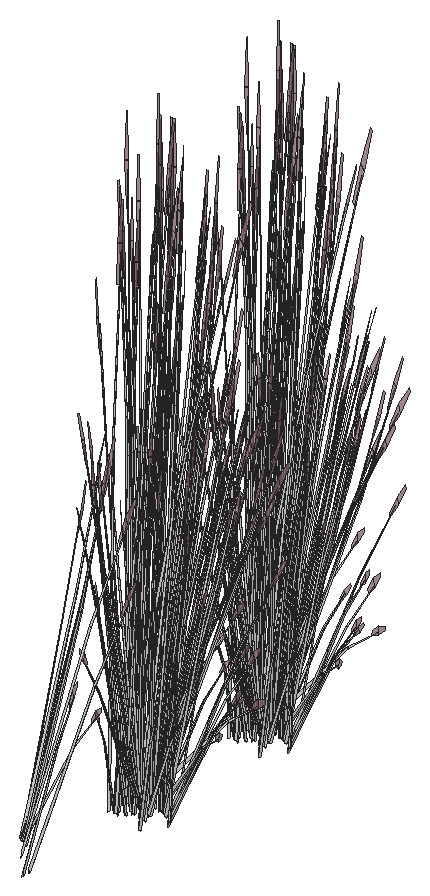
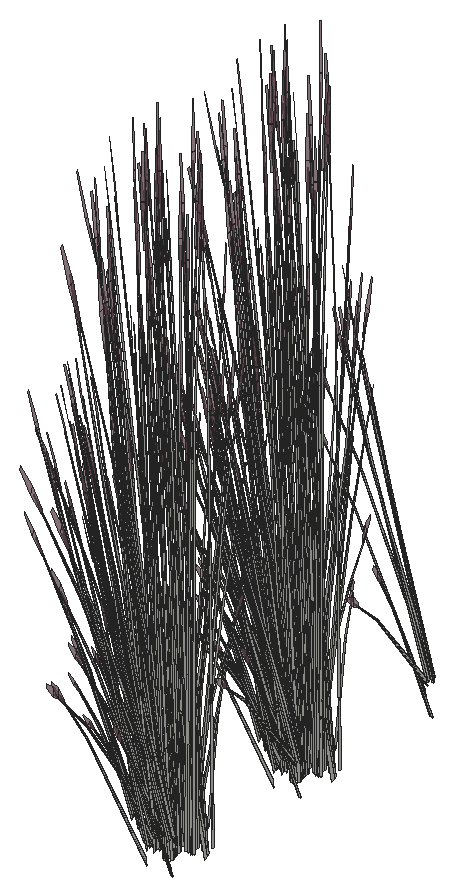
# SketchUp Ruby script. Lengths in inches.
U = 1.inch
M = Sketchup.active_model
def pt(a) = Geom::Point3d.new(a.map { |v| v * U })
def face(e, loops, mat)
  f = e.add_face(loops[0].map { |a| pt(a) })
  loops[1..].each { |l| e.add_face(l.map { |a| pt(a) }).erase! }
  f.material = f.back_material = mat if mat
  f
end
# faces: each face lists its corners as indices into pts; further lists are holes
def faces(e, pts, list, mat = nil) = list.each { |f| face(e, (f[0].is_a?(Array) ? f : [f]).map { |l| l.map { |i| pts[i] } }, mat) }
# xy, xz, yz: faces in a plane at the given z, y or x. An outline is a flat list of corners, or four numbers for a rectangle; further outlines are holes
def ring(l) = l.size == 4 ? [[l[0], l[1]], [l[2], l[1]], [l[2], l[3]], [l[0], l[3]]] : l.each_slice(2).to_a
def flat(e, list, mat, &to3) = list.each { |f| face(e, (f[0].is_a?(Array) ? f : [f]).map { |l| ring(l).map { |u, v| to3.(u, v) } }, mat) }
def xy(e, z, list, mat = nil) = flat(e, list, mat) { |x, y| [x, y, z] }
def xz(e, y, list, mat = nil) = flat(e, list, mat) { |x, z| [x, y, z] }
def yz(e, x, list, mat = nil) = flat(e, list, mat) { |y, z| [x, y, z] }
def lines(e, pts, list) = list.each { |a, b| e.add_line(pt(pts[a]), pt(pts[b])) }
# prism: a flat outline (further loops are holes) pulled along v
def prism(e, loops, v, mat = nil)
  f = face(e, loops, mat); d = Geom::Vector3d.new(v.map { |x| x * U })
  f.pushpull(f.normal.samedirection?(d) ? d.length : -d.length)
end
def box(e, o, s, mat = nil) = prism(e, [[o, [o[0] + s[0], o[1], o[2]], [o[0] + s[0], o[1] + s[1], o[2]], [o[0], o[1] + s[1], o[2]]]], [0, 0, s[2]], mat)
def at(x, y, z, deg = 0) = Geom::Transformation.translation(pt([x, y, z])) * Geom::Transformation.rotation(ORIGIN, Z_AXIS, deg.degrees)
def axes(o, x, y, z) = Geom::Transformation.new([*x, 0, *y, 0, *z, 0, *pt(o).to_a, 1])
def part(name) = M.definitions.add(name)
# library, detail: a bought-in or finely detailed component or shape, given as its bounding box
def library(name, o, s) = part(name).tap { |d| box(d.entities, o, s) }
def detail(e, o, s) = box(e.add_group.entities, o, s)
def put(e, d, t, mat = nil) = e.add_instance(d, t).tap { |i| i.material = mat if mat }
def group(e, t, mat = nil) = e.add_group.tap { |g| g.transformation = t; g.material = mat if mat }.entities
root = M.entities
M.materials.add("LightPink_Translucent").color = [144, 107, 117]
M.materials["LightPink_Translucent"].alpha = 0.75
c1 = part("blade")
p = [[2.15,0.21,22],[0,0.17,0],[0.09,0.45,0],[2.18,0.31,22],[2.29,0.31,22],[0.38,0.45,0],
  [2.48,0.24,33],[2.49,0.24,33],[2.48,0.22,33]]
faces(c1.entities,p,[[0,1,2,3],[4,5,2,3],[6,3,4,7],[8,0,3,6]])
c2 = part("seeds")
p = [[0.3,-0.1,1.38],[-0.01,-0.03,1.59],[-0.01,-0.03,0.03],[0.14,-0.07,-0.07],[0.29,-0.03,3],[0.15,0.01,3.11]]
faces(c2.entities,p,[[0,1,2,3],[1,0,4,5]],"LightPink_Translucent")
c3 = part("blade with seeds")
put(c3.entities,c1,at(0,0,0))
put(c3.entities,c2,axes([2.4,0.25,30.99],[1.5799,-0.05474,1.17369],[-0.12525,1.92788,0.29478],[-0.07173,-0.02425,1.56792]))
put(root,c3,axes([342.66,137.39,656.125],[0.00872,-0.13732,1.17261],[0.41669,-0.15339,-0.25218],[0.12863,0.16436,0.50135]))
put(root,c3,axes([341.53,137.87,658.13],[0.48353,-0.19287,-0.09971],[0.23761,0.34232,-0.55346],[0.0638,0.14425,0.84097]))
put(root,c3,axes([341.61,137.95,655.22],[0.07997,-0.02254,1.44601],[0.48102,0.12407,-0.2209],[0.01407,0.13984,0.2463]))
put(root,c3,axes([341.94,137.86,657.84],[0.48573,0.10385,-0.41901],[-0.16649,0.35605,-0.32456],[0.04454,0.14335,0.80174]))
put(root,c3,axes([342.22,137.12,657.18],[-0.11295,-0.13301,1.40529],[0.52192,-0.11198,0.11363],[0.11796,0.20881,0.60075]))
put(root,c3,axes([341.72,138.07,657.71],[-0.14896,0.31857,-0.29039],[-0.4346,-0.09292,0.3749],[0.03985,0.12826,0.71734]))
put(root,c3,axes([341.77,137.79,658.08],[0.23583,0.33684,-0.58257],[-0.48546,0.18772,0.0703],[0.05515,0.16275,0.8241]))
put(root,c3,axes([341.41,138.64,657.87],[0.06263,0.06671,1.43454],[0.50546,0.02621,-0.22687],[0.05083,0.14712,0.11505]))
put(root,c3,axes([343.01,147.42,656.125],[-0.14045,0.08385,1.17261],[-0.42064,-0.14676,-0.25218],[0.07797,-0.18252,0.50135]))
put(root,c3,axes([343.35,148.04,658.08],[0.01286,-0.38319,-0.58257],[0.54141,0.02574,0.0703],[0.05714,-0.16234,0.8241]))
put(root,c3,axes([344.11,147.4375,657.87],[-0.00477,-0.08245,1.43454],[-0.40285,-0.23829,-0.22687],[0.06228,-0.14445,0.11505]))
put(root,c3,axes([342.74,147.84,657.18],[-0.092,0.14239,1.40529],[-0.38596,-0.29467,0.11363],[0.17411,-0.18366,0.60075]))
put(root,c3,axes([344,147.14,657.86],[-0.05018,0.03164,1.45454],[-0.49165,-0.10676,-0.13744],[-0.0178,-0.13809,0.2574]))
put(root,c3,axes([342.49,146.75,656.27],[0.06339,0.24157,0.94186],[-0.35163,-0.13379,0.69201],[0.03784,-0.12369,0.20745]))
put(root,c3,axes([343.24,147.91,657.84],[-0.35372,-0.27835,-0.41901],[0.37366,-0.24377,-0.32456],[0.05382,-0.14142,0.80174]))
put(root,c3,axes([342.47,147.5,657.88],[0.48688,0.1083,0.39362],[-0.16649,0.35605,0.32456],[-0.02926,-0.14002,0.8145]))
put(root,c3,axes([343.61,148.06,658.13],[-0.54305,-0.02053,-0.09971],[0.01484,-0.38862,-0.55346],[0.03772,-0.14967,0.84097]))
put(root,c3,axes([343.57,147.81,657.71],[0.33433,-0.21811,-0.29039],[0.31649,0.24905,0.3749],[0.04815,-0.12654,0.71734]))
put(root,c3,axes([342.6,147.47,657.88],[0.36409,-0.14079,0.05273],[0.17821,0.25674,0.41509],[-0.03516,-0.11317,0.63295]))
put(root,c3,axes([343.99,147.67,655.22],[-0.07396,-0.03263,1.44601],[-0.18997,-0.3646,-0.2209],[0.12815,-0.09894,0.2463]))
put(root,c3,axes([343.57,147.89,657.88],[0.35185,0.28265,0.39362],[-0.37366,0.24377,0.32456],[0.0649,-0.13261,0.8145]))
put(root,c3,axes([343.7,147.92,657.88],[0.40605,0.0193,0.05273],[-0.01113,0.29147,0.41509],[0.04249,-0.11165,0.63295]))
put(root,c3,axes([343.4,148.12,658.14],[-0.33433,0.21811,0.29039],[-0.31649,-0.24905,-0.3749],[0.04815,-0.12654,0.71734]))
put(root,c3,axes([343.99,148.7,658.08],[0.2581,-0.32687,-0.58257],[0.45228,0.2323,0.0703],[0.15411,-0.11843,0.8241]))
put(root,c3,axes([341.2,147.75,655.95],[-0.30893,-0.41511,0],[0.51685,-0.2315,-0.42318],[0.11772,-0.05273,1.34243]))
put(root,c3,axes([343.98,148.55,657.84],[-0.12693,-0.37826,-0.41901],[0.48071,-0.06617,-0.32456],[0.13776,-0.1016,0.80174]))
put(root,c3,axes([344.2,148.82,658.13],[-0.45707,-0.22842,-0.09971],[0.26332,-0.3308,-0.55346],[0.12913,-0.11499,0.84097]))
put(root,c3,axes([341.62,147.6875,655.65],[0.46245,-0.20713,-0.40713],[0.27641,0.37142,0],[0.10533,-0.04718,1.29153]))
put(root,c3,axes([344.36,148.4,656.125],[-0.17652,-0.01227,1.17261],[-0.18084,-0.32916,-0.25218],[0.21685,-0.09312,0.50135]))
put(root,c3,axes([345.33,148.72,657.86],[-0.06454,-0.00315,1.45454],[-0.268,-0.33712,-0.13744],[0.10763,-0.11085,0.2574]))
put(root,c3,axes([342.17,148.54,655.6875],[0.33282,-0.31137,-0.51129],[0.41344,0.28235,-0.13419],[0.13336,-0.07767,1.12859]))
put(root,c3,axes([344.57,147.8,656.27],[-0.16458,0.21088,0.94186],[-0.14146,-0.28332,0.69201],[0.13593,-0.07099,0.20745]))
put(root,c3,axes([344.33,148.59,657.71],[0.43011,-0.0592,-0.29039],[0.11357,0.33844,0.3749],[0.12326,-0.0909,0.71734]))
put(root,c3,axes([341.59,149.08,655.8125],[0.23974,-0.37328,-0.36686],[0.49814,0.17965,0.17656],[0,-0.08605,1.17788]))
put(root,c3,axes([341.81,148.9,656.1875],[-0.05758,-0.4727,-0.23858],[0.59969,-0.02858,-0.41002],[0.1056,-0.06296,1.3096]))
put(root,c3,axes([343.98,148.79,658.14],[-0.43011,0.0592,0.29039],[-0.11357,-0.33844,-0.3749],[0.12326,-0.0909,0.71734]))
put(root,c3,axes([341.73,147.85,655.66],[0.46099,0.1025,-0.25402],[-0.11607,0.36097,0.25402],[0.09293,-0.04163,1.13959]))
put(root,c3,axes([344.37,148.74,657.88],[0.33921,0.17422,0.05273],[-0.19749,0.2481,0.41509],[0.10876,-0.08021,0.63295]))
put(root,c3,axes([344.27,148.66,657.88],[0.12254,0.38127,0.39362],[-0.48071,0.06617,0.32456],[0.14168,-0.08967,0.8145]))
put(root,c3,axes([345.57,149.125,657.87],[0.06857,-0.0631,1.43454],[-0.08776,-0.38707,-0.22687],[0.17204,-0.07339,0.11505]))
put(root,c3,axes([341.88,149.27,656],[0.55674,0.20078,0.19733],[-0.26794,0.4172,0.41002],[0,-0.09617,1.31645]))
put(root,c3,axes([341.7,148.99,656.23],[-0.53657,0.02557,0.36686],[-0.04852,-0.4245,-0.17656],[0.09606,-0.04302,1.17788]))
put(root,c3,axes([344.22,149.71,658.13],[-0.24861,-0.37512,-0.09971],[0.44125,-0.18434,-0.55346],[0.18594,-0.04949,0.84097]))
put(root,c3,axes([344.2,149.39,657.84],[0.13386,-0.37682,-0.41901],[0.45895,0.12916,-0.32456],[0.18478,-0.03455,0.80174]))
put(root,c3,axes([343.47,147.86,655.95],[0.30893,-0.41511,0],[0.51685,0.2315,-0.42318],[0.11772,0.05273,1.34243]))
put(root,c3,axes([341.69,149.14,655.9375],[0.21483,0.46323,0.37519],[-0.61383,0.16108,0.14723],[0.0075,-0.08512,1.30262]))
put(root,c3,axes([344.6875,149.5,655.625],[-0.31825,0.04971,1.16098],[-0.05066,-0.39572,0.06645],[0.2229,-0.0599,0.66064]))
put(root,c3,axes([345.27,149.15,655.85],[-0.30634,-0.2649,-0.0532],[0.33551,-0.24272,-0.24121],[0.09507,-0.01709,0.7956]))
put(root,c3,axes([342.46,149.18,655.81],[0,-0.47933,0],[0.61786,0,0],[0,0,1.47154]))
put(root,c3,axes([343.21,148.07,656.03],[-0.46245,-0.20713,0.40713],[0.27641,-0.37142,0],[0.10533,0.04718,1.29153]))
put(root,c3,axes([344.11,149.53,658.08],[0.43419,-0.18296,-0.58257],[0.24197,0.37661,0.0703],[0.20979,-0.04278,0.8241]))
put(root,c3,axes([342.17,148.88,655.9375],[-0.40969,0.37595,0.37519],[-0.48673,-0.33186,0.14723],[0.09877,-0.03752,1.30262]))
put(root,c3,axes([341.45,148.26,656.03],[-0.14274,0.41171,0.14467],[-0.52234,-0.11651,0.28771],[0.09023,-0.00201,1.31534]))
put(root,c3,axes([344.05,149.6,658.14],[-0.41064,-0.11557,0.29039],[0.11977,-0.33716,-0.3749],[0.16533,-0.03092,0.71734]))
put(root,c3,axes([341.24,148.59,655.31],[-0.48636,0.16585,1.05721],[-0.1548,-0.47588,0.41079],[0.29865,0.00792,1.20246]))
put(root,c3,axes([342.54,148.72,656.15],[0.09532,-0.36971,0.11873],[0.46572,0.06418,-0.33905],[0.08476,0.03796,1.0393]))
put(root,c3,axes([345.04,149.24,655.22],[-0.02582,-0.06289,1.44601],[0.17911,-0.36789,-0.2209],[0.18067,-0.00529,0.2463]))
put(root,c3,axes([342.35,148.8125,656.23],[-0.29683,-0.34771,0.36686],[0.44961,-0.24485,-0.17656],[0.09606,0.04302,1.17788]))
put(root,c3,axes([342.5,148.84,656.1875],[0.49889,-0.27503,-0.23858],[0.33175,0.38862,-0.41002],[0.12309,0.03947,1.3096]))
put(root,c3,axes([344.48,149.5625,657.71],[0.41064,0.11557,-0.29039],[-0.11977,0.33716,0.3749],[0.16533,-0.03092,0.71734]))
put(root,c3,axes([343.75,148.11,655.65],[0.46245,0.20713,-0.40713],[-0.27641,0.37142,0],[0.10533,0.04718,1.29153]))
put(root,c3,axes([342.88,149.29,655.81],[0.55282,0,0],[0,0.42888,0],[0,0,1.46294]))
put(root,c3,axes([343.03,148.28,656.03],[-0.53096,0.10995,0.14467],[-0.13111,-0.40919,0.28771],[0.04735,0.05962,1.31534]))
put(root,c3,axes([343.36,149.14,657.18],[-0.20495,0.00938,1.40529],[0.13596,-0.40664,0.11363],[0.29207,0.02515,0.60075]))
put(root,c3,axes([343.625,148.26,655.66],[0.11607,0.36097,-0.25402],[-0.46099,0.1025,0.25402],[0.09293,0.04163,1.13959]))
put(root,c3,axes([344.42,149.7,657.88],[0.18148,0.28246,0.05273],[-0.33093,0.13825,0.41509],[0.14588,-0.02728,0.63295]))
put(root,c3,axes([342.7,149.07,655.95],[-0.62452,-0.08728,0.40343],[0.1271,-0.49295,0.15831],[0.09127,0.0476,1.40067]))
put(root,c3,axes([344.39,149.6,657.88],[-0.1396,0.37772,0.39362],[-0.45895,-0.12916,0.32456],[0.18049,-0.0227,0.8145]))
put(root,c3,axes([342.2,150.29,655.81],[-0.16122,-0.35715,0],[0.46037,-0.12507,0],[0,0,1.26584]))
put(root,c3,axes([342.8,150.24,655.79],[0.51876,-0.14056,-0.15742],[0.18228,0.40489,0.00007],[0.05726,-0.01554,1.42596]))
put(root,c3,axes([342.87,149.47,655.82],[0.34492,0.26758,0],[-0.34492,0.26758,0],[0,0,1.38798]))
put(root,c3,axes([343.8,149.35,656.03],[-0.38822,-0.30175,0.14467],[0.39123,-0.29268,0.28771],[-0.04288,0.06162,1.31534]))
put(root,c3,axes([343.08,148.9,655.6875],[0.514,0.06792,-0.51129],[-0.10846,0.41895,-0.13419],[0.15339,0.05076,1.12859]))
put(root,c3,axes([345.35,149.63,656.27],[-0.30529,0.06839,0.94186],[0.1437,-0.28265,0.69201],[0.16196,0.01934,0.20745]))
put(root,c3,axes([342.86,149.16,656.23],[0.23974,-0.37328,0.36686],[0.49814,0.17965,-0.17656],[0,0.08605,1.17788]))
put(root,c3,axes([345.21,150.83,657.86],[-0.04468,-0.03627,1.45454],[0.09773,-0.38875,-0.13744],[0.17599,-0.02484,0.2574]))
put(root,c3,axes([342.77,149.37,655.88],[0,0.4791,-0.04622],[-0.61786,0,0],[0,0.01506,1.47081]))
put(root,c3,axes([342.8125,149.03,655.8125],[0.29683,0.34771,-0.36686],[-0.44961,0.24485,0.17656],[0.09606,0.04302,1.17788]))
put(root,c3,axes([344.82,150.5,657.22],[-0.09457,-0.34824,-0.02863],[0.44699,-0.08006,-0.12982],[0.09334,0.02208,0.42819]))
put(root,c3,axes([343.66,150.49,658.13],[0.02646,-0.4213,-0.09971],[0.50094,0.01152,-0.55346],[0.19293,0.02926,0.84097]))
put(root,c3,axes([344.12,149.37,656.03],[0,-0.41426,0.40713],[0.55282,0,0],[0,0.09435,1.29153]))
put(root,c3,axes([343.07,149.24,656.15],[0.46037,-0.12081,0.11873],[0.16122,0.34498,-0.33905],[0,0.07592,1.0393]))
put(root,c3,axes([343.59,150.33,658.14],[-0.28114,-0.25937,0.29039],[0.32102,-0.24553,-0.3749],[0.16311,0.03736,0.71734]))
put(root,c3,axes([344.78,150.08,656.125],[-0.119,-0.10189,1.17261],[0.15483,-0.33705,-0.25218],[0.24077,0.04566,0.50135]))
put(root,c3,axes([342.65,150.46,655.81],[0.49814,0.18599,0],[-0.23974,0.38645,0],[0,0,1.43462]))
put(root,c3,axes([344.1,150.24,657.87],[0.106,-0.00701,1.43454],[0.29074,-0.32184,-0.22687],[0.18854,0.04248,0.11505]))
put(root,c3,axes([343.6875,150.29,658.08],[0.49394,0.00997,-0.58257],[-0.03317,0.42002,0.0703],[0.20925,0.04433,0.8241]))
put(root,c3,axes([342.47,150.3,655.88],[0.21483,0.47591,-0.0493],[-0.61383,0.16676,0],[0.0075,0.01662,1.41182]))
put(root,c3,axes([344.49,149.4375,655.95],[0.61786,0,0],[0,0.463,-0.42318],[0,0.10545,1.34243]))
put(root,c3,axes([344.25,149.67,655.8],[-0.61756,-0.00331,-0.04081],[0,-0.463,0.40953],[-0.01941,0.1054,1.29849]))
put(root,c3,axes([342.91,149.27,656.1875],[0.55647,0.19766,-0.23858],[-0.26794,0.4172,-0.41002],[0.01749,0.10243,1.3096]))
put(root,c3,axes([343.98,150.46,657.71],[0.28114,0.25937,-0.29039],[-0.32102,0.24553,0.3749],[0.16311,0.03736,0.71734]))
put(root,c3,axes([344.12,149.74,655.66],[-0.34492,0.25847,-0.25402],[-0.34492,-0.25847,0.25402],[0,0.08325,1.13959]))
put(root,c3,axes([343.84,150.5625,657.88],[-0.02488,0.31501,0.05273],[-0.3757,-0.00864,0.41509],[0.14392,0.03296,0.63295]))
put(root,c3,axes([342.85,149.58,655.8125],[-0.23974,0.37328,-0.36686],[-0.49814,-0.17965,0.17656],[0,0.08605,1.17788]))
put(root,c3,axes([343.875,150.46,657.88],[-0.36434,0.27297,0.39362],[-0.31422,-0.28988,0.32456],[0.17094,0.05035,0.8145]))
put(root,c3,axes([342.72,150.78,658.14],[-0.07631,-0.33368,0.29039],[0.43626,-0.08811,-0.3749],[0.11718,0.09562,0.71734]))
put(root,c3,axes([344.36,149.75,655.65],[0,0.41426,-0.40713],[-0.55282,0,0],[0,0.09435,1.29153]))
put(root,c3,axes([342.97,149.8,657.18],[-0.18354,-0.07137,1.40529],[0.37983,-0.29943,0.11363],[0.23673,0.13508,0.60075]))
put(root,c3,axes([343.01,148.86,657.67],[-0.42697,-0.21524,1.13392],[0.45084,-0.33512,0.48925],[0.13776,0.20196,1.09604]))
put(root,c3,axes([343.65,150.61,656.27],[-0.27821,-0.11912,0.94186],[0.35924,-0.12103,0.69201],[0.09689,0.10252,0.20745]))
put(root,c3,axes([342.68,150.95,658.13],[0.29444,-0.35459,-0.09971],[0.4264,0.20428,-0.55346],[0.14822,0.10018,0.84097]))
put(root,c3,axes([342.29,151.24,657.86],[0.00146,-0.05015,1.45454],[0.42344,-0.22127,-0.13744],[0.14708,0.07898,0.2574]))
put(root,c3,axes([343.73,151.05,655.22],[0.036,-0.05981,1.44601],[0.45322,-0.17614,-0.2209],[0.1374,0.09116,0.2463]))
put(root,c3,axes([343.13,149.69,655.72],[0.18118,0.37929,-0.56754],[-0.52191,0.1366,-0.14895],[0.02003,0.12844,1.25274]))
put(root,c3,axes([343.03,150.77,657.84],[0.48758,-0.09847,-0.41901],[0.08529,0.37293,-0.32456],[0.13096,0.10687,0.80174]))
put(root,c3,axes([341.67,150.83,658.14],[0.14896,-0.31857,0.29039],[0.4346,0.09292,-0.3749],[0.03985,0.12826,0.71734]))
put(root,c3,axes([343.7,151.15,656.1875],[-0.31686,-0.01299,0.86149],[0.20925,-0.27594,0.47565],[0.12517,0.09804,0.67577]))
put(root,c3,axes([342.79,151.08,657.88],[-0.22457,0.26316,0.05273],[-0.3198,-0.15321,0.41509],[0.10339,0.08437,0.63295]))
put(root,c3,axes([342.26,151.97,658.63],[0.34145,-0.23766,-0.0532],[0.31287,0.26029,-0.24121],[0.02203,0.07375,0.7956]))
put(root,c3,axes([342.88,151.01,657.88],[-0.49145,0.09507,0.39362],[-0.08529,-0.37293,0.32456],[0.11558,0.10991,0.8145]))
put(root,c3,axes([342.66,150.48,656.125],[0.00872,-0.13732,1.17261],[0.41669,-0.15339,-0.25218],[0.12863,0.16436,0.50135]))
put(root,c3,axes([341.53,150.96,658.13],[0.48353,-0.19287,-0.09971],[0.23761,0.34232,-0.55346],[0.0638,0.14425,0.84097]))
put(root,c3,axes([341.61,151.04,655.22],[0.07997,-0.02254,1.44601],[0.48102,0.12407,-0.2209],[0.01407,0.13984,0.2463]))
put(root,c3,axes([341.94,150.95,657.84],[0.48573,0.10385,-0.41901],[-0.16649,0.35605,-0.32456],[0.04454,0.14335,0.80174]))
put(root,c3,axes([342.22,150.21,657.18],[-0.11295,-0.13301,1.40529],[0.52192,-0.11198,0.11363],[0.11796,0.20881,0.60075]))
put(root,c3,axes([341.72,151.17,657.71],[-0.14896,0.31857,-0.29039],[-0.4346,-0.09292,0.3749],[0.03985,0.12826,0.71734]))
put(root,c3,axes([341.77,150.88,658.08],[0.23583,0.33684,-0.58257],[-0.48546,0.18772,0.0703],[0.05515,0.16275,0.8241]))
put(root,c3,axes([341.41,151.73,657.87],[0.06263,0.06671,1.43454],[0.50546,0.02621,-0.22687],[0.05083,0.14712,0.11505]))
put(root,c3,axes([343.01,160.05,656.125],[-0.14045,0.08385,1.17261],[-0.42064,-0.14676,-0.25218],[0.07797,-0.18252,0.50135]))
put(root,c3,axes([343.35,160.67,658.08],[0.01286,-0.38319,-0.58257],[0.54141,0.02574,0.0703],[0.05714,-0.16234,0.8241]))
put(root,c3,axes([344.11,160.08,657.87],[-0.00477,-0.08245,1.43454],[-0.40285,-0.23829,-0.22687],[0.06228,-0.14445,0.11505]))
put(root,c3,axes([342.41,160.06,657.71],[0.14896,-0.31857,-0.29039],[0.4346,0.09292,0.3749],[-0.03985,-0.12826,0.71734]))
put(root,c3,axes([342.74,160.48,657.18],[-0.092,0.14239,1.40529],[-0.38596,-0.29467,0.11363],[0.17411,-0.18366,0.60075]))
put(root,c3,axes([344,159.78,657.86],[-0.05018,0.03164,1.45454],[-0.49165,-0.10676,-0.13744],[-0.0178,-0.13809,0.2574]))
put(root,c3,axes([342.49,159.39,656.27],[0.06339,0.24157,0.94186],[-0.35163,-0.13379,0.69201],[0.03784,-0.12369,0.20745]))
put(root,c3,axes([343.24,160.55,657.84],[-0.35372,-0.27835,-0.41901],[0.37366,-0.24377,-0.32456],[0.05382,-0.14142,0.80174]))
put(root,c3,axes([342.47,160.13,657.88],[0.48688,0.1083,0.39362],[-0.16649,0.35605,0.32456],[-0.02926,-0.14002,0.8145]))
put(root,c3,axes([343.61,160.69,658.13],[-0.54305,-0.02053,-0.09971],[0.01484,-0.38862,-0.55346],[0.03772,-0.14967,0.84097]))
put(root,c3,axes([343.57,160.44,657.71],[0.33433,-0.21811,-0.29039],[0.31649,0.24905,0.3749],[0.04815,-0.12654,0.71734]))
put(root,c3,axes([342.6,160.11,657.88],[0.36409,-0.14079,0.05273],[0.17821,0.25674,0.41509],[-0.03516,-0.11317,0.63295]))
put(root,c3,axes([343.99,160.3125,655.22],[-0.07396,-0.03263,1.44601],[-0.18997,-0.3646,-0.2209],[0.12815,-0.09894,0.2463]))
put(root,c3,axes([343.57,160.53,657.88],[0.35185,0.28265,0.39362],[-0.37366,0.24377,0.32456],[0.0649,-0.13261,0.8145]))
put(root,c3,axes([343.7,160.56,657.88],[0.40605,0.0193,0.05273],[-0.01113,0.29147,0.41509],[0.04249,-0.11165,0.63295]))
put(root,c3,axes([343.4,160.75,658.14],[-0.33433,0.21811,0.29039],[-0.31649,-0.24905,-0.3749],[0.04815,-0.12654,0.71734]))
put(root,c3,axes([343.99,161.34,658.08],[0.2581,-0.32687,-0.58257],[0.45228,0.2323,0.0703],[0.15411,-0.11843,0.8241]))
put(root,c3,axes([341.2,160.39,655.95],[-0.30893,-0.41511,0],[0.51685,-0.2315,-0.42318],[0.11772,-0.05273,1.34243]))
put(root,c3,axes([343.98,161.1875,657.84],[-0.12693,-0.37826,-0.41901],[0.48071,-0.06617,-0.32456],[0.13776,-0.1016,0.80174]))
put(root,c3,axes([344.2,161.46,658.13],[-0.45707,-0.22842,-0.09971],[0.26332,-0.3308,-0.55346],[0.12913,-0.11499,0.84097]))
put(root,c3,axes([341.62,160.33,655.65],[0.46245,-0.20713,-0.40713],[0.27641,0.37142,0],[0.10533,-0.04718,1.29153]))
put(root,c3,axes([344.36,161.04,656.125],[-0.17652,-0.01227,1.17261],[-0.18084,-0.32916,-0.25218],[0.21685,-0.09312,0.50135]))
put(root,c3,axes([345.33,161.36,657.86],[-0.06454,-0.00315,1.45454],[-0.268,-0.33712,-0.13744],[0.10763,-0.11085,0.2574]))
put(root,c3,axes([342.17,161.17,655.6875],[0.33282,-0.31137,-0.51129],[0.41344,0.28235,-0.13419],[0.13336,-0.07767,1.12859]))
put(root,c3,axes([344.57,160.4375,656.27],[-0.16458,0.21088,0.94186],[-0.14146,-0.28332,0.69201],[0.13593,-0.07099,0.20745]))
put(root,c3,axes([344.33,161.23,657.71],[0.43011,-0.0592,-0.29039],[0.11357,0.33844,0.3749],[0.12326,-0.0909,0.71734]))
put(root,c3,axes([341.59,161.72,655.8125],[0.23974,-0.37328,-0.36686],[0.49814,0.17965,0.17656],[0,-0.08605,1.17788]))
put(root,c3,axes([341.81,161.54,656.1875],[-0.05758,-0.4727,-0.23858],[0.59969,-0.02858,-0.41002],[0.1056,-0.06296,1.3096]))
put(root,c3,axes([343.98,161.43,658.14],[-0.43011,0.0592,0.29039],[-0.11357,-0.33844,-0.3749],[0.12326,-0.0909,0.71734]))
put(root,c3,axes([341.73,160.49,655.66],[0.46099,0.1025,-0.25402],[-0.11607,0.36097,0.25402],[0.09293,-0.04163,1.13959]))
put(root,c3,axes([344.37,161.375,657.88],[0.33921,0.17422,0.05273],[-0.19749,0.2481,0.41509],[0.10876,-0.08021,0.63295]))
put(root,c3,axes([344.27,161.3,657.88],[0.12254,0.38127,0.39362],[-0.48071,0.06617,0.32456],[0.14168,-0.08967,0.8145]))
put(root,c3,axes([345.57,161.76,657.87],[0.06857,-0.0631,1.43454],[-0.08776,-0.38707,-0.22687],[0.17204,-0.07339,0.11505]))
put(root,c3,axes([341.88,161.91,656],[0.55674,0.20078,0.19733],[-0.26794,0.4172,0.41002],[0,-0.09617,1.31645]))
put(root,c3,axes([341.7,161.625,656.23],[-0.53657,0.02557,0.36686],[-0.04852,-0.4245,-0.17656],[0.09606,-0.04302,1.17788]))
put(root,c3,axes([344.22,162.35,658.13],[-0.24861,-0.37512,-0.09971],[0.44125,-0.18434,-0.55346],[0.18594,-0.04949,0.84097]))
put(root,c3,axes([344.2,162.03,657.84],[0.13386,-0.37682,-0.41901],[0.45895,0.12916,-0.32456],[0.18478,-0.03455,0.80174]))
put(root,c3,axes([343.47,160.49,655.95],[0.30893,-0.41511,0],[0.51685,0.2315,-0.42318],[0.11772,0.05273,1.34243]))
put(root,c3,axes([341.69,161.78,655.9375],[0.21483,0.46323,0.37519],[-0.61383,0.16108,0.14723],[0.0075,-0.08512,1.30262]))
put(root,c3,axes([344.6875,162.13,655.625],[-0.31825,0.04971,1.16098],[-0.05066,-0.39572,0.06645],[0.2229,-0.0599,0.66064]))
put(root,c3,axes([345.27,161.78,655.85],[-0.30634,-0.2649,-0.0532],[0.33551,-0.24272,-0.24121],[0.09507,-0.01709,0.7956]))
put(root,c3,axes([342.46,161.82,655.81],[0,-0.47933,0],[0.61786,0,0],[0,0,1.47154]))
put(root,c3,axes([343.21,160.71,656.03],[-0.46245,-0.20713,0.40713],[0.27641,-0.37142,0],[0.10533,0.04718,1.29153]))
put(root,c3,axes([344.11,162.17,658.08],[0.43419,-0.18296,-0.58257],[0.24197,0.37661,0.0703],[0.20979,-0.04278,0.8241]))
put(root,c3,axes([342.17,161.52,655.9375],[-0.40969,0.37595,0.37519],[-0.48673,-0.33186,0.14723],[0.09877,-0.03752,1.30262]))
put(root,c3,axes([341.45,160.9,656.03],[-0.14274,0.41171,0.14467],[-0.52234,-0.11651,0.28771],[0.09023,-0.00201,1.31534]))
put(root,c3,axes([344.05,162.24,658.14],[-0.41064,-0.11557,0.29039],[0.11977,-0.33716,-0.3749],[0.16533,-0.03092,0.71734]))
put(root,c3,axes([341.24,161.23,655.31],[-0.48636,0.16585,1.05721],[-0.1548,-0.47588,0.41079],[0.29865,0.00792,1.20246]))
put(root,c3,axes([342.54,161.36,656.15],[0.09532,-0.36971,0.11873],[0.46572,0.06418,-0.33905],[0.08476,0.03796,1.0393]))
put(root,c3,axes([345.04,161.875,655.22],[-0.02582,-0.06289,1.44601],[0.17911,-0.36789,-0.2209],[0.18067,-0.00529,0.2463]))
put(root,c3,axes([342.35,161.45,656.23],[-0.29683,-0.34771,0.36686],[0.44961,-0.24485,-0.17656],[0.09606,0.04302,1.17788]))
put(root,c3,axes([342.5,161.48,656.1875],[0.49889,-0.27503,-0.23858],[0.33175,0.38862,-0.41002],[0.12309,0.03947,1.3096]))
put(root,c3,axes([344.48,162.2,657.71],[0.41064,0.11557,-0.29039],[-0.11977,0.33716,0.3749],[0.16533,-0.03092,0.71734]))
put(root,c3,axes([343.75,160.74,655.65],[0.46245,0.20713,-0.40713],[-0.27641,0.37142,0],[0.10533,0.04718,1.29153]))
put(root,c3,axes([342.88,161.93,655.81],[0.55282,0,0],[0,0.42888,0],[0,0,1.46294]))
put(root,c3,axes([343.03,160.92,656.03],[-0.53096,0.10995,0.14467],[-0.13111,-0.40919,0.28771],[0.04735,0.05962,1.31534]))
put(root,c3,axes([343.36,161.78,657.18],[-0.20495,0.00938,1.40529],[0.13596,-0.40664,0.11363],[0.29207,0.02515,0.60075]))
put(root,c3,axes([343.625,160.9,655.66],[0.11607,0.36097,-0.25402],[-0.46099,0.1025,0.25402],[0.09293,0.04163,1.13959]))
put(root,c3,axes([344.42,162.34,657.88],[0.18148,0.28246,0.05273],[-0.33093,0.13825,0.41509],[0.14588,-0.02728,0.63295]))
put(root,c3,axes([342.7,161.71,655.95],[-0.62452,-0.08728,0.40343],[0.1271,-0.49295,0.15831],[0.09127,0.0476,1.40067]))
put(root,c3,axes([344.39,162.24,657.88],[-0.1396,0.37772,0.39362],[-0.45895,-0.12916,0.32456],[0.18049,-0.0227,0.8145]))
put(root,c3,axes([342.2,162.92,655.81],[-0.16122,-0.35715,0],[0.46037,-0.12507,0],[0,0,1.26584]))
put(root,c3,axes([342.8,162.875,655.79],[0.51876,-0.14056,-0.15742],[0.18228,0.40489,0.00007],[0.05726,-0.01554,1.42596]))
put(root,c3,axes([342.87,162.11,655.82],[0.34492,0.26758,0],[-0.34492,0.26758,0],[0,0,1.38798]))
put(root,c3,axes([343.8,161.99,656.03],[-0.38822,-0.30175,0.14467],[0.39123,-0.29268,0.28771],[-0.04288,0.06162,1.31534]))
put(root,c3,axes([343.08,161.54,655.6875],[0.514,0.06792,-0.51129],[-0.10846,0.41895,-0.13419],[0.15339,0.05076,1.12859]))
put(root,c3,axes([345.35,162.27,656.27],[-0.30529,0.06839,0.94186],[0.1437,-0.28265,0.69201],[0.16196,0.01934,0.20745]))
put(root,c3,axes([342.86,161.8,656.23],[0.23974,-0.37328,0.36686],[0.49814,0.17965,-0.17656],[0,0.08605,1.17788]))
put(root,c3,axes([345.21,163.46,657.86],[-0.04468,-0.03627,1.45454],[0.09773,-0.38875,-0.13744],[0.17599,-0.02484,0.2574]))
put(root,c3,axes([342.77,162.01,655.88],[0,0.4791,-0.04622],[-0.61786,0,0],[0,0.01506,1.47081]))
put(root,c3,axes([342.8125,161.67,655.8125],[0.29683,0.34771,-0.36686],[-0.44961,0.24485,0.17656],[0.09606,0.04302,1.17788]))
put(root,c3,axes([344.82,163.14,657.22],[-0.09457,-0.34824,-0.02863],[0.44699,-0.08006,-0.12982],[0.09334,0.02208,0.42819]))
put(root,c3,axes([343.66,163.13,658.13],[0.02646,-0.4213,-0.09971],[0.50094,0.01152,-0.55346],[0.19293,0.02926,0.84097]))
put(root,c3,axes([344.12,162,656.03],[0,-0.41426,0.40713],[0.55282,0,0],[0,0.09435,1.29153]))
put(root,c3,axes([343.07,161.88,656.15],[0.46037,-0.12081,0.11873],[0.16122,0.34498,-0.33905],[0,0.07592,1.0393]))
put(root,c3,axes([343.59,162.96,658.14],[-0.28114,-0.25937,0.29039],[0.32102,-0.24553,-0.3749],[0.16311,0.03736,0.71734]))
put(root,c3,axes([344.78,162.72,656.125],[-0.119,-0.10189,1.17261],[0.15483,-0.33705,-0.25218],[0.24077,0.04566,0.50135]))
put(root,c3,axes([342.65,163.09,655.81],[0.49814,0.18599,0],[-0.23974,0.38645,0],[0,0,1.43462]))
put(root,c3,axes([344.1,162.88,657.87],[0.106,-0.00701,1.43454],[0.29074,-0.32184,-0.22687],[0.18854,0.04248,0.11505]))
put(root,c3,axes([343.6875,162.93,658.08],[0.49394,0.00997,-0.58257],[-0.03317,0.42002,0.0703],[0.20925,0.04433,0.8241]))
put(root,c3,axes([342.47,162.9375,655.88],[0.21483,0.47591,-0.0493],[-0.61383,0.16676,0],[0.0075,0.01662,1.41182]))
put(root,c3,axes([344.49,162.07,655.95],[0.61786,0,0],[0,0.463,-0.42318],[0,0.10545,1.34243]))
put(root,c3,axes([344.25,162.3125,655.8],[-0.61756,-0.00331,-0.04081],[0,-0.463,0.40953],[-0.01941,0.1054,1.29849]))
put(root,c3,axes([342.91,161.91,656.1875],[0.55647,0.19766,-0.23858],[-0.26794,0.4172,-0.41002],[0.01749,0.10243,1.3096]))
put(root,c3,axes([343.98,163.1,657.71],[0.28114,0.25937,-0.29039],[-0.32102,0.24553,0.3749],[0.16311,0.03736,0.71734]))
put(root,c3,axes([344.12,162.38,655.66],[-0.34492,0.25847,-0.25402],[-0.34492,-0.25847,0.25402],[0,0.08325,1.13959]))
put(root,c3,axes([343.84,163.2,657.88],[-0.02488,0.31501,0.05273],[-0.3757,-0.00864,0.41509],[0.14392,0.03296,0.63295]))
put(root,c3,axes([342.85,162.22,655.8125],[-0.23974,0.37328,-0.36686],[-0.49814,-0.17965,0.17656],[0,0.08605,1.17788]))
put(root,c3,axes([343.875,163.1,657.88],[-0.36434,0.27297,0.39362],[-0.31422,-0.28988,0.32456],[0.17094,0.05035,0.8145]))
put(root,c3,axes([342.72,163.42,658.14],[-0.07631,-0.33368,0.29039],[0.43626,-0.08811,-0.3749],[0.11718,0.09562,0.71734]))
put(root,c3,axes([344.36,162.39,655.65],[0,0.41426,-0.40713],[-0.55282,0,0],[0,0.09435,1.29153]))
put(root,c3,axes([342.97,162.4375,657.18],[-0.18354,-0.07137,1.40529],[0.37983,-0.29943,0.11363],[0.23673,0.13508,0.60075]))
put(root,c3,axes([343.01,161.5,657.67],[-0.42697,-0.21524,1.13392],[0.45084,-0.33512,0.48925],[0.13776,0.20196,1.09604]))
put(root,c3,axes([343.65,163.25,656.27],[-0.27821,-0.11912,0.94186],[0.35924,-0.12103,0.69201],[0.09689,0.10252,0.20745]))
put(root,c3,axes([342.68,163.59,658.13],[0.29444,-0.35459,-0.09971],[0.4264,0.20428,-0.55346],[0.14822,0.10018,0.84097]))
put(root,c3,axes([342.29,163.88,657.86],[0.00146,-0.05015,1.45454],[0.42344,-0.22127,-0.13744],[0.14708,0.07898,0.2574]))
put(root,c3,axes([343.73,163.69,655.22],[0.036,-0.05981,1.44601],[0.45322,-0.17614,-0.2209],[0.1374,0.09116,0.2463]))
put(root,c3,axes([343.13,162.33,655.72],[0.18118,0.37929,-0.56754],[-0.52191,0.1366,-0.14895],[0.02003,0.12844,1.25274]))
put(root,c3,axes([343.03,163.41,657.84],[0.48758,-0.09847,-0.41901],[0.08529,0.37293,-0.32456],[0.13096,0.10687,0.80174]))
put(root,c3,axes([341.67,163.47,658.14],[0.14896,-0.31857,0.29039],[0.4346,0.09292,-0.3749],[0.03985,0.12826,0.71734]))
put(root,c3,axes([343.7,163.79,656.1875],[-0.31686,-0.01299,0.86149],[0.20925,-0.27594,0.47565],[0.12517,0.09804,0.67577]))
put(root,c3,axes([342.79,163.72,657.88],[-0.22457,0.26316,0.05273],[-0.3198,-0.15321,0.41509],[0.10339,0.08437,0.63295]))
put(root,c3,axes([342.26,164.6,658.63],[0.34145,-0.23766,-0.0532],[0.31287,0.26029,-0.24121],[0.02203,0.07375,0.7956]))
put(root,c3,axes([342.88,163.64,657.88],[-0.49145,0.09507,0.39362],[-0.08529,-0.37293,0.32456],[0.11558,0.10991,0.8145]))
put(root,c3,axes([342.66,163.12,656.125],[0.00872,-0.13732,1.17261],[0.41669,-0.15339,-0.25218],[0.12863,0.16436,0.50135]))
put(root,c3,axes([341.53,163.6,658.13],[0.48353,-0.19287,-0.09971],[0.23761,0.34232,-0.55346],[0.0638,0.14425,0.84097]))
put(root,c3,axes([341.61,163.68,655.22],[0.07997,-0.02254,1.44601],[0.48102,0.12407,-0.2209],[0.01407,0.13984,0.2463]))
put(root,c3,axes([341.94,163.59,657.84],[0.48573,0.10385,-0.41901],[-0.16649,0.35605,-0.32456],[0.04454,0.14335,0.80174]))
put(root,c3,axes([342.22,162.85,657.18],[-0.11295,-0.13301,1.40529],[0.52192,-0.11198,0.11363],[0.11796,0.20881,0.60075]))
